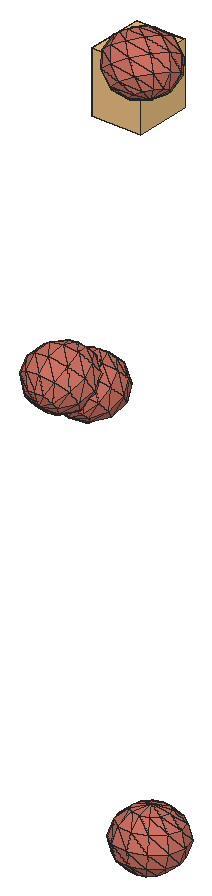
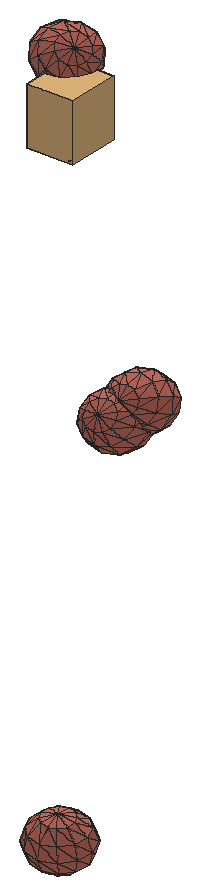
# SketchUp Ruby script. Lengths in inches.
U = 1.inch
M = Sketchup.active_model
def pt(a) = Geom::Point3d.new(a.map { |v| v * U })
def face(e, loops, mat)
  f = e.add_face(loops[0].map { |a| pt(a) })
  loops[1..].each { |l| e.add_face(l.map { |a| pt(a) }).erase! }
  f.material = f.back_material = mat if mat
  f
end
# faces: each face lists its corners as indices into pts; further lists are holes
def faces(e, pts, list, mat = nil) = list.each { |f| face(e, (f[0].is_a?(Array) ? f : [f]).map { |l| l.map { |i| pts[i] } }, mat) }
# xy, xz, yz: faces in a plane at the given z, y or x. An outline is a flat list of corners, or four numbers for a rectangle; further outlines are holes
def ring(l) = l.size == 4 ? [[l[0], l[1]], [l[2], l[1]], [l[2], l[3]], [l[0], l[3]]] : l.each_slice(2).to_a
def flat(e, list, mat, &to3) = list.each { |f| face(e, (f[0].is_a?(Array) ? f : [f]).map { |l| ring(l).map { |u, v| to3.(u, v) } }, mat) }
def xy(e, z, list, mat = nil) = flat(e, list, mat) { |x, y| [x, y, z] }
def xz(e, y, list, mat = nil) = flat(e, list, mat) { |x, z| [x, y, z] }
def yz(e, x, list, mat = nil) = flat(e, list, mat) { |y, z| [x, y, z] }
def lines(e, pts, list) = list.each { |a, b| e.add_line(pt(pts[a]), pt(pts[b])) }
# prism: a flat outline (further loops are holes) pulled along v
def prism(e, loops, v, mat = nil)
  f = face(e, loops, mat); d = Geom::Vector3d.new(v.map { |x| x * U })
  f.pushpull(f.normal.samedirection?(d) ? d.length : -d.length)
end
def box(e, o, s, mat = nil) = prism(e, [[o, [o[0] + s[0], o[1], o[2]], [o[0] + s[0], o[1] + s[1], o[2]], [o[0], o[1] + s[1], o[2]]]], [0, 0, s[2]], mat)
def at(x, y, z, deg = 0) = Geom::Transformation.translation(pt([x, y, z])) * Geom::Transformation.rotation(ORIGIN, Z_AXIS, deg.degrees)
def axes(o, x, y, z) = Geom::Transformation.new([*x, 0, *y, 0, *z, 0, *pt(o).to_a, 1])
def part(name) = M.definitions.add(name)
# library, detail: a bought-in or finely detailed component or shape, given as its bounding box
def library(name, o, s) = part(name).tap { |d| box(d.entities, o, s) }
def detail(e, o, s) = box(e.add_group.entities, o, s)
def put(e, d, t, mat = nil) = e.add_instance(d, t).tap { |i| i.material = mat if mat }
def group(e, t, mat = nil) = e.add_group.tap { |g| g.transformation = t; g.material = mat if mat }.entities
root = M.entities
M.materials.add("green").color = [174, 139, 102]
M.materials.add("vio").color = [206, 114, 100]
c1 = part("3DGeom~194_Defintion")
p = [[111.52,-262.8,-376.52],[-124.92,-186.52,-431.46],[-6.51,0,-500],[214.07,-101.27,-435.87],[-225.34,101.27,-430.15],[113.66,186.52,-434.56],
  [-121.28,262.8,-373.49],[318.08,-268.67,-220.68],[318.08,-268.67,-220.68],[377.29,-175.41,-254.95],[377.29,-175.41,-254.95],[318.13,60.26,-379.2],
  [318.13,60.26,-379.2],[318.13,60.26,-379.2],[203.36,323.0625,-252.6875],[-43.59,381.05,-215.98],[-43.59,381.05,-215.98],[203.36,323.0625,-252.6875],
  [37.95,-381.05,-217.04],[-209.87,-323.0625,-247.3125],[37.95,-381.05,-217.04],[-327.89,-60.26,-370.8],[-327.89,-60.26,-370.8],[-383.79,175.41,-245.05],
  [-225.34,101.27,-430.15],[-383.79,175.41,-245.05],[-323.71,268.67,-212.33],[-323.71,268.67,-212.33],[377.29,-175.41,-254.95],[318.13,60.26,-379.2],
  [437.37,-82.15,-222.23],[437.37,-82.15,-222.23],[318.13,60.26,-379.2],[395.82,178.51,-221.69],[318.13,60.26,-379.2],[203.36,323.0625,-252.6875],
  [395.82,178.51,-221.69],[275.6,-336.9375,-128.61],[37.95,-381.05,-217.04],[111.52,-262.8,-376.52],[275.6,-336.9375,-128.61],[111.52,-262.8,-376.52],
  [318.08,-268.67,-220.68],[-121.28,262.8,-373.49],[-323.71,268.67,-212.33],[-278.86,336.9375,-121.39],[-121.28,262.8,-373.49],[-43.59,381.05,-215.98],
  [-401.46,-178.51,-211.32],[-401.46,-178.51,-211.32],[-443,82.15,-210.78],[-327.89,-60.26,-370.8],[-327.89,-60.26,-370.8],[-383.79,175.41,-245.05],
  [318.08,-268.67,-220.68],[377.29,-175.41,-254.95],[439.41,-202.54,-5.72],[203.36,323.0625,-252.6875],[238.58,373.04,-3.1],[203.36,323.0625,-252.6875],
  [-13.09,424.33,0.17],[203.36,323.0625,-252.6875],[238.58,373.04,-3.1],[13.09,-424.33,-0.17],[-238.58,-373.04,3.1],[-209.87,-323.0625,-247.3125],
  [-209.87,-323.0625,-247.3125],[-238.58,-373.04,3.1],[-401.46,-178.51,-211.32],[-209.87,-323.0625,-247.3125],[-383.79,175.41,-245.05],[-439.41,202.54,5.72],
  [-323.71,268.67,-212.33],[-383.79,175.41,-245.05],[482.22,-13.88,-131.3],[426.32,221.79,-5.55],[275.6,-336.9375,-128.61],[261.25,-361.93,-3.4],
  [261.25,-361.93,-3.4],[275.6,-336.9375,-128.61],[-261.25,361.93,3.4],[-278.86,336.9375,-121.39],[-323.71,268.67,-212.33],[-238.58,-373.04,3.1],
  [-426.32,-221.79,5.55],[-401.46,-178.51,-211.32],[-485.47,13.88,-118.7],[-401.46,-178.51,-211.32],[-401.46,-178.51,-211.32],[499.83,11.11,-6.5],
  [261.25,-361.93,-3.4],[-261.25,361.93,3.4],[-278.86,336.9375,-121.39],[-499.83,-11.11,6.5],[485.47,-13.88,118.7],[401.46,178.51,211.32],
  [278.86,-336.9375,121.39],[323.71,-268.67,212.33],[383.79,-175.41,245.05],[443,-82.15,210.78],[209.87,323.0625,247.3125],[209.87,323.0625,247.3125],
  [278.86,-336.9375,121.39],[261.25,-361.93,-3.4],[238.58,373.04,-3.1],[-37.95,381.05,217.04],[209.87,323.0625,247.3125],[238.58,373.04,-3.1],
  [-37.95,381.05,217.04],[43.59,-381.05,215.98],[278.86,-336.9375,121.39],[-275.6,336.9375,128.61],[-37.95,381.05,217.04],[-203.36,-323.0625,252.6875],
  [-203.36,-323.0625,252.6875],[-238.58,-373.04,3.1],[-275.6,336.9375,128.61],[-261.25,361.93,3.4],[-203.36,-323.0625,252.6875],[-395.82,-178.51,221.69],
  [-482.22,13.88,131.3],[-437.37,82.15,222.23],[-377.29,175.41,254.95],[-377.29,175.41,254.95],[-318.08,268.67,220.68],[-318.08,268.67,220.68],
  [-275.6,336.9375,128.61],[327.89,60.26,370.8],[323.71,-268.67,212.33],[278.86,-336.9375,121.39],[-37.95,381.05,217.04],[-318.08,268.67,220.68],
  [-318.13,-60.26,379.2],[-318.13,-60.26,379.2],[225.34,-101.27,430.15],[225.34,-101.27,430.15],[401.46,178.51,211.32],[124.92,186.52,431.46],
  [327.89,60.26,370.8],[401.46,178.51,211.32],[209.87,323.0625,247.3125],[323.71,-268.67,212.33],[121.28,-262.8,373.49],[383.79,-175.41,245.05],
  [121.28,-262.8,373.49],[323.71,-268.67,212.33],[121.28,-262.8,373.49],[-203.36,-323.0625,252.6875],[43.59,-381.05,215.98],[-37.95,381.05,217.04],
  [-318.08,268.67,220.68],[-111.52,262.8,376.51],[-37.95,381.05,217.04],[-111.52,262.8,376.51],[-318.08,268.67,220.68],[-377.29,175.41,254.95],
  [-113.66,-186.52,434.56],[-395.82,-178.51,221.69],[-203.36,-323.0625,252.6875],[-318.13,-60.26,379.2],[-395.82,-178.51,221.69],[-214.07,101.27,435.87],
  [-437.37,82.15,222.23],[-437.37,82.15,222.23],[383.79,-175.41,245.05],[225.34,-101.27,430.15],[121.28,-262.8,373.49],[121.28,-262.8,373.49],
  [-203.36,-323.0625,252.6875],[327.89,60.26,370.8],[6.51,0,500],[327.89,60.26,370.8],[121.28,-262.8,373.49]]
faces(c1.entities,p,[[0,1,2],[0,2,3],[1,4,2],[3,2,5],[2,4,6],[2,6,5],[7,0,3],[8,3,9],
  [10,3,11],[3,5,12],[13,5,14],[5,6,15],[5,16,17],[18,19,1],[20,1,0],[19,21,1],
  [1,21,4],[22,23,24],[4,25,26],[4,27,6],[28,29,30],[31,32,33],[34,35,36],[37,38,39],
  [40,41,42],[43,44,45],[46,45,47],[19,48,21],[49,50,51],[52,50,53],[54,55,56],[55,31,56],
  [33,57,58],[59,47,60],[61,60,62],[63,64,65],[63,66,38],[67,68,69],[70,50,71],[72,73,71],
  [31,74,56],[31,33,74],[74,33,75],[33,58,75],[76,54,56],[77,63,38],[78,38,79],[47,45,80],
  [47,80,60],[81,82,71],[83,84,85],[84,86,87],[88,86,50],[50,86,71],[74,89,56],[74,75,89],
  [90,76,56],[91,92,71],[84,93,86],[86,93,71],[89,94,56],[89,95,94],[89,75,95],[96,90,56],
  [97,96,56],[98,97,56],[99,98,56],[94,99,56],[75,100,95],[75,58,101],[102,63,103],[104,105,106],
  [107,60,108],[109,64,63],[110,109,63],[60,80,111],[60,111,112],[109,113,64],[114,84,115],[116,117,71],
  [118,119,84],[119,93,84],[93,120,71],[120,121,71],[121,122,71],[123,124,71],[125,126,71],[119,120,93],
  [94,127,99],[94,95,127],[128,109,129],[130,111,131],[132,120,119],[133,121,120],[99,134,98],[99,127,135],
  [136,137,138],[139,140,137],[141,142,109],[143,144,145],[146,147,148],[149,150,151],[140,152,153],[153,154,155],
  [156,157,158],[156,159,160],[161,162,159],[161,155,163],[164,165,166],[140,153,137],[167,156,168],[153,155,161],
  [169,170,165],[171,137,170],[165,156,172],[137,153,161],[170,159,156],[170,161,159],[165,170,156],[137,161,170]],"vio")
c2 = part("3DGeom~189_Defintion")
p = [[117.375,12.85,-489.11],[33.19,-268.35,-390.125],[-76.27,-85.37,-487.14],[256.79,-154.93,-392.4],[251.43,147.02,-400.02],[-53.49,177.1875,-454.76],
  [23.91,254.65,-403.32],[-199.3,-309.86,-283.32],[-277.61,-121.32,-394.64],[-165.29,120.48,-453.62],[-210.02,294.05,-298.55],[-281.54,99.72,-400.21],
  [46.16,332.12,-313.1],[-281.54,99.72,-400.21],[-277.61,-121.32,-394.64],[-432.71,-85.37,-236.39],[-281.54,99.72,-400.21],[-371.08,120.48,-308.85],
  [-371.08,120.48,-308.85],[411.58,0,-289.54],[289.98,281.2,-243.75],[411.58,0,-289.54],[251.43,147.02,-400.02],[289.98,281.2,-243.75],
  [-277.61,-121.32,-394.64],[-199.3,-309.86,-283.32],[-378.39,-268.35,-100.59],[-277.61,-121.32,-394.64],[133.75,-379.42,-188.58],[327.4,-281.2,-190.55],
  [133.75,-379.42,-188.58],[411.58,0,-289.54],[327.4,-281.2,-190.55],[256.79,-154.93,-392.4],[33.19,-268.35,-390.125],[-67.59,-415.375,-96.08],
  [-199.3,-309.86,-283.32],[33.19,-268.35,-390.125],[133.75,-379.42,-188.58],[7.3125,388.83,-208.26],[289.98,281.2,-243.75],[46.16,332.12,-313.1],
  [46.16,332.12,-313.1],[-210.02,294.05,-298.55],[-500,12.85,-54.8],[-409.93,177.1875,-204.01],[-210.02,294.05,-298.55],[-387.68,254.65,-113.79],
  [-210.02,294.05,-298.55],[-387.68,254.65,-113.79],[-310.28,332.12,-62.35],[-210.02,294.05,-298.55],[-198.48,388.83,-63.49],[-210.02,294.05,-298.55],
  [-82.23,409.58,-116.9],[-210.02,294.05,-298.55],[-210.02,294.05,-298.55],[411.58,0,-289.54],[461.45,-147.02,-101.47],[327.4,-281.2,-190.55],
  [456.09,154.93,-109.09],[411.58,0,-289.54],[289.98,281.2,-243.75],[411.58,0,-289.54],[-199.3,-309.86,-283.32],[-222.6875,-379.42,62.16],
  [-199.3,-309.86,-283.32],[-222.6875,-379.42,62.16],[-378.39,-268.35,-100.59],[222.6875,379.42,-62.16],[289.98,281.2,-243.75],[222.6875,379.42,-62.16],
  [289.98,281.2,-243.75],[-456.09,-154.93,109.09],[-461.45,147.02,101.47],[-387.68,254.65,-113.79],[327.4,-281.2,-190.55],[198.48,-388.83,63.49],
  [327.4,-281.2,-190.55],[310.28,-332.12,62.35],[310.28,-332.12,62.35],[327.4,-281.2,-190.55],[82.23,-409.58,116.9],[67.59,415.375,96.08],
  [-387.68,254.65,-113.79],[-327.4,281.2,190.55],[-387.68,254.65,-113.79],[-327.4,281.2,190.55],[-310.28,332.12,-62.35],[500,-12.85,54.8],
  [378.39,268.35,100.59],[222.6875,379.42,-62.16],[387.68,-254.65,113.79],[310.28,-332.12,62.35],[-222.6875,-379.42,62.16],[-289.98,-281.2,243.75],
  [-7.3125,-388.83,208.26],[-222.6875,-379.42,62.16],[-133.75,379.42,188.58],[-327.4,281.2,190.55],[378.39,268.35,100.59],[-411.58,0,289.54],
  [409.93,-177.1875,204.01],[432.71,85.37,236.39],[-222.6875,-379.42,62.16],[-46.16,-332.12,313.1],[-222.6875,-379.42,62.16],[-46.16,-332.12,313.1],
  [-289.98,-281.2,243.75],[210.02,-294.05,298.55],[387.68,-254.65,113.79],[199.3,309.86,283.32],[378.39,268.35,100.59],[199.3,309.86,283.32],
  [-256.79,154.93,392.4],[-256.79,154.93,392.4],[-327.4,281.2,190.55],[-251.43,-147.02,400.02],[-251.43,-147.02,400.02],[210.02,-294.05,298.55],
  [-327.4,281.2,190.55],[-33.19,268.35,390.13],[-133.75,379.42,188.58],[-33.19,268.35,390.13],[-327.4,281.2,190.55],[-256.79,154.93,392.4],
  [-33.19,268.35,390.13],[371.08,-120.48,308.85],[210.02,-294.05,298.55],[-46.16,-332.12,313.1],[277.61,121.32,394.64],[199.3,309.86,283.32],
  [-289.98,-281.2,243.75],[-46.16,-332.12,313.1],[-23.91,-254.65,403.32],[-289.98,-281.2,243.75],[-251.43,-147.02,400.02],[-33.19,268.35,390.13],
  [277.61,121.32,394.64],[199.3,309.86,283.32],[-411.58,0,289.54],[-117.375,-12.85,489.11],[-411.58,0,289.54],[210.02,-294.05,298.55],
  [53.49,-177.1875,454.76],[210.02,-294.05,298.55],[165.29,-120.48,453.62],[210.02,-294.05,298.55],[281.54,-99.72,400.21],[210.02,-294.05,298.55],
  [371.08,-120.48,308.85],[281.54,-99.72,400.21],[210.02,-294.05,298.55],[281.54,-99.72,400.21],[76.27,85.37,487.14],[-33.19,268.35,390.13],
  [-33.19,268.35,390.13],[277.61,121.32,394.64],[281.54,-99.72,400.21],[277.61,121.32,394.64],[281.54,-99.72,400.21]]
faces(c2.entities,p,[[0,1,2],[0,3,1],[4,3,0],[5,0,2],[6,0,5],[6,4,0],[2,7,8],[2,1,7],
  [9,2,8],[5,2,9],[5,9,10],[6,5,10],[9,8,11],[9,11,10],[12,4,6],[12,6,10],
  [13,14,15],[16,15,17],[11,18,10],[4,19,3],[20,21,22],[12,23,4],[24,25,26],[27,26,15],
  [3,28,1],[3,29,30],[31,32,33],[34,35,36],[37,38,35],[39,40,41],[39,42,43],[17,15,44],
  [17,44,45],[17,45,46],[45,47,48],[49,50,51],[50,52,53],[54,39,55],[52,54,56],[57,58,59],
  [60,58,61],[62,60,63],[64,35,65],[66,67,68],[69,60,70],[39,71,72],[15,26,73],[15,73,44],
  [54,71,39],[45,44,74],[45,74,75],[76,77,38],[78,79,77],[58,80,81],[38,82,35],[38,77,82],
  [54,83,71],[52,83,54],[84,74,85],[86,87,88],[60,89,58],[90,89,60],[91,90,60],[58,92,93],
  [89,92,58],[26,94,95],[26,95,73],[35,96,97],[35,82,96],[50,98,52],[52,98,83],[50,99,98],
  [83,100,71],[44,73,101],[44,101,74],[89,102,92],[103,102,89],[90,103,89],[104,96,105],[106,107,108],
  [77,79,109],[79,110,109],[82,77,109],[83,111,112],[98,111,83],[113,103,90],[74,101,114],[74,115,116],
  [73,95,117],[73,118,101],[92,102,119],[96,82,109],[120,121,122],[98,123,111],[124,125,126],[102,127,128],
  [103,127,102],[129,96,109],[130,127,103],[131,130,103],[132,133,134],[135,134,136],[137,138,139],[140,136,141],
  [142,141,125],[134,133,143],[144,134,145],[146,144,147],[148,146,149],[150,151,152],[130,153,127],[125,154,155],
  [156,154,157],[125,141,154],[154,158,159],[136,134,144],[136,144,141],[154,146,160],[141,144,146],[141,146,154]],"vio")
c3 = part("3DGeom~224_Defintion")
p = [[81.72,-275.8,-371.94],[-133.11,-167.42,-440.41],[24.02,0,-500],[217.8,-130.81,-423.55],[-176.2,130.81,-442.48],[217.8,-130.81,-423.55],
  [174.72,167.42,-425.62],[-45.69,275.8,-378.0625],[-312.28,-14.1875,-390.87],[-329.21,226.5625,-266.39],[-253.86,310.28,-229.2],[-253.86,310.28,-229.2],
  [-23.47,-381.94,-218.13],[-254.58,-289.99,-262.81],[-23.47,-381.94,-218.13],[217.8,-130.81,-423.55],[348.3125,14.1875,-359.13],[348.3125,14.1875,-359.13],
  [278.6,289.99,-237.19],[44.27,381.94,-214.88],[44.27,381.94,-214.88],[278.6,289.99,-237.19],[274.66,-310.28,-203.8125],[217.8,-130.81,-423.55],
  [274.66,-310.28,-203.8125],[217.8,-130.81,-423.55],[353.23,-226.5625,-233.61],[353.23,-226.5625,-233.61],[217.8,-130.81,-423.55],[348.3125,14.1875,-359.13],
  [-417.47,-120.33,-237.0625],[-417.47,-120.33,-237.0625],[-407.77,142.85,-236.59],[-312.28,-14.1875,-390.87],[-407.77,142.85,-236.59],[-45.69,275.8,-378.0625],
  [-253.86,310.28,-229.2],[-201.92,371.56,-134.99],[-45.69,275.8,-378.0625],[44.27,381.94,-214.88],[213.93,-371.56,-115.01],[-23.47,-381.94,-218.13],
  [81.72,-275.8,-371.94],[213.93,-371.56,-115.01],[81.72,-275.8,-371.94],[274.66,-310.28,-203.8125],[428.58,-142.85,-196.42],[438.28,120.33,-195.95],
  [348.3125,14.1875,-359.13],[278.6,289.99,-237.19],[438.28,120.33,-195.95],[-329.21,226.5625,-266.39],[-407.77,142.85,-236.59],[-394.01,261.61,-18.93],
  [-253.86,310.28,-229.2],[-329.21,226.5625,-266.39],[-69.59,-420.79,-3.34],[-307.83,-334.85,-14.79],[-254.58,-289.99,-262.81],[-254.58,-289.99,-262.81],
  [-307.83,-334.85,-14.79],[-417.47,-120.33,-237.0625],[-254.58,-289.99,-262.81],[278.6,289.99,-237.19],[307.83,334.85,14.79],[278.6,289.99,-237.19],
  [69.59,420.79,3.34],[278.6,289.99,-237.19],[307.83,334.85,14.79],[-307.83,-334.85,-14.79],[-463.59,-159.18,-22.27],[-417.47,-120.33,-237.0625],
  [-468.51,81.57,-147.8],[-417.47,-120.33,-237.0625],[-417.47,-120.33,-237.0625],[-407.77,142.85,-236.59],[-407.77,142.85,-236.59],[274.66,-310.28,-203.8125],
  [394.01,-261.61,18.93],[394.01,-261.61,18.93],[-201.92,371.56,-134.99],[-253.86,310.28,-229.2],[187.3,-393.99,9],[213.93,-371.56,-115.01],
  [-187.3,393.99,-9],[213.93,-371.56,-115.01],[394.01,-261.61,18.93],[480.52,-81.57,-102.2],[394.01,-261.61,18.93],[463.59,159.18,22.27],
  [-495.13,59.14,-23.79],[-394.01,261.61,-18.93],[213.93,-371.56,-115.01],[394.01,-261.61,18.93],[495.13,-59.14,23.79],[394.01,-261.61,18.93],
  [-438.28,-120.33,195.95],[-480.52,81.57,102.2],[-278.6,-289.99,237.19],[-307.83,-334.85,-14.79],[-278.6,-289.99,237.19],[-428.58,142.85,196.42],
  [-353.23,226.5625,233.61],[-274.66,310.28,203.8125],[-274.66,310.28,203.8125],[-213.93,371.56,115.01],[-213.93,371.56,115.01],[-394.01,261.61,-18.93],
  [-44.27,-381.94,214.88],[-278.6,-289.99,237.19],[201.92,-371.56,134.99],[307.83,334.85,14.79],[23.47,381.94,218.13],[23.47,381.94,218.13],
  [254.58,289.99,262.81],[307.83,334.85,14.79],[23.47,381.94,218.13],[254.58,289.99,262.81],[253.86,-310.28,229.2],[201.92,-371.56,134.99],
  [394.01,-261.61,18.93],[329.21,-226.5625,266.39],[394.01,-261.61,18.93],[407.77,-142.85,236.59],[394.01,-261.61,18.93],[468.51,-81.57,147.8],
  [394.01,-261.61,18.93],[394.01,-261.61,18.93],[417.47,120.33,237.0625],[254.58,289.99,262.81],[-348.3125,-14.1875,359.13],[-348.3125,-14.1875,359.13],
  [23.47,381.94,218.13],[-274.66,310.28,203.8125],[253.86,-310.28,229.2],[312.28,14.1875,390.87],[312.28,14.1875,390.87],[-174.72,-167.42,425.62],
  [-438.28,-120.33,195.95],[-278.6,-289.99,237.19],[-348.3125,-14.1875,359.13],[-438.28,-120.33,195.95],[-217.8,130.81,423.55],[-348.3125,-14.1875,359.13],
  [-217.8,130.81,423.55],[-81.72,275.8,371.94],[-274.66,310.28,203.8125],[-353.23,226.5625,233.61],[23.47,381.94,218.13],[-274.66,310.28,203.8125],
  [-81.72,275.8,371.94],[45.69,-275.8,378.0625],[-278.6,-289.99,237.19],[-44.27,-381.94,214.88],[253.86,-310.28,229.2],[45.69,-275.8,378.0625],
  [254.58,289.99,262.81],[23.47,381.94,218.13],[329.21,-226.5625,266.39],[45.69,-275.8,378.0625],[253.86,-310.28,229.2],[-353.23,226.5625,233.61],
  [-217.8,130.81,423.55],[407.77,-142.85,236.59],[176.2,-130.81,442.48],[329.21,-226.5625,266.39],[407.77,-142.85,236.59],[312.28,14.1875,390.87],
  [417.47,120.33,237.0625],[133.11,167.42,440.41],[417.47,120.33,237.0625],[45.69,-275.8,378.0625],[-278.6,-289.99,237.19],[329.21,-226.5625,266.39],
  [45.69,-275.8,378.0625],[-24.02,0,500],[45.69,-275.8,378.0625]]
faces(c3.entities,p,[[0,1,2],[0,2,3],[1,4,2],[5,2,6],[2,4,7],[2,7,6],[1,8,4],[8,9,4],
  [4,9,10],[4,11,7],[12,13,1],[14,1,0],[13,8,1],[15,6,16],[17,6,18],[6,7,19],
  [6,20,21],[22,0,23],[24,25,26],[27,28,29],[13,30,8],[31,32,33],[8,34,9],[35,36,37],
  [38,37,39],[40,41,42],[43,44,45],[27,29,46],[46,29,47],[48,49,50],[51,52,53],[54,55,53],
  [56,57,58],[56,59,41],[60,61,62],[47,63,64],[65,39,66],[67,66,68],[69,70,71],[70,72,73],
  [74,72,75],[76,72,53],[77,27,78],[27,46,79],[80,81,53],[82,56,41],[82,41,83],[39,37,84],
  [39,84,66],[85,77,86],[46,87,88],[46,47,87],[87,47,89],[47,64,89],[70,90,72],[72,90,53],
  [84,37,91],[82,92,93],[87,94,95],[87,89,94],[96,90,70],[96,97,90],[90,97,53],[98,70,99],
  [100,96,70],[97,101,53],[101,102,53],[102,103,53],[104,105,53],[106,84,107],[108,57,56],[108,109,57],
  [66,84,106],[110,108,56],[110,56,82],[111,66,112],[66,106,113],[110,82,93],[89,64,114],[115,116,117],
  [118,119,120],[121,118,122],[123,121,124],[125,123,126],[94,125,127],[94,89,128],[89,129,128],[94,128,125],
  [130,97,96],[131,101,97],[132,106,133],[134,108,110],[125,135,123],[125,128,136],[137,138,139],[137,140,141],
  [142,101,143],[144,102,101],[145,146,147],[148,149,150],[151,152,153],[154,155,108],[156,157,145],[158,159,160],
  [145,161,162],[163,164,165],[166,167,164],[168,169,167],[170,156,169],[171,137,172],[156,145,169],[173,164,174],
  [175,140,137],[175,162,140],[169,145,162],[164,137,176],[167,175,164],[167,169,175],[169,162,175],[164,175,137]],"vio")
c4 = library("3DGeom~9_Defintion",[-447.05,-500,-392.82],[894.1,1000,785.64])
c5 = part("3DGeom~10_Defintion")
p = [[-376.65,-477.04,-383.86],[-408.2,-455.37,-392.67],[-389.75,-464.73,-392.82],[-376.65,-477.04,-383.86],[-442.82,-474.42,-333.72],[-408.2,-455.37,-392.67],
  [-408.2,-455.37,-392.67],[-442.82,-474.42,-333.72],[-441.29,-454.05,-367.6],[-408.2,-455.37,-392.67],[-441.29,-454.05,-367.6],[-427.07,-451.46,-383.43],
  [-378.18,-497.41,-349.98],[-442.82,-474.42,-333.72],[-376.65,-477.04,-383.86],[-378.18,-497.41,-349.98],[-376.65,-477.04,-383.86],[-372.41,-489,-368.18],
  [-442.82,-474.42,-333.72],[-447.05,-462.46,-349.4],[-441.29,-454.05,-367.6],[-411.26,-496.09,-324.91],[-378.18,-497.41,-349.98],[-392.4,-500,-334.15],
  [-411.26,-496.09,-324.91],[-442.82,-474.42,-333.72],[-378.18,-497.41,-349.98],[-442.82,-474.42,-333.72],[-411.26,-496.09,-324.91],[-429.72,-486.73,-324.76],
  [401.4,485.85,384.88],[441.04,458.37,319.44],[429.72,472.35,311.5],[401.4,485.85,384.88],[429.72,472.35,311.5],[416.12,486.26,314.46],
  [401.4,485.85,384.88],[416.12,486.26,314.46],[403.89,496.38,327.52],[401.4,485.85,384.88],[447.05,448.07,336.15],[441.04,458.37,319.44],
  [401.4,485.85,384.88],[403.89,496.38,327.52],[396.3,500,347.18],[401.4,485.85,384.88],[446.15,444.22,357.14],[447.05,448.07,336.15],
  [401.4,485.85,384.88],[396.3,500,347.18],[395.39,496.14,368.18],[401.4,485.85,384.88],[438.56,447.84,376.81],[446.15,444.22,357.14],
  [401.4,485.85,384.88],[426.33,457.96,389.87],[438.56,447.84,376.81],[401.4,485.85,384.88],[412.73,471.87,392.82],[426.33,457.96,389.87]]
faces(c5.entities,p,[[0,1,2],[3,4,5],[6,7,8],[9,10,11],[12,13,14],[15,16,17],[18,19,20],[21,22,23],
  [24,25,26],[27,28,29],[30,31,32],[33,34,35],[36,37,38],[39,40,41],[42,43,44],[45,46,47],
  [48,49,50],[51,52,53],[54,55,56],[57,58,59]],"green")
c6 = part("3DGeom~192_Defintion")
p = [[46.59,-12.33,-500],[-151.08,-242.85,-384.34],[-208.06,-36.06,-455.29],[69.45,-222.31,-423.06],[288.76,14.69,-410.73],[11.25,200.94,-442.97],
  [220.97,224.35,-365.66],[-323.33,-255.02,-239.97],[-406.96,-50.11,-288.59],[-323.33,-255.02,-239.97],[-209.29,180.4,-404.25],[-406.96,-50.11,-288.59],
  [-27.11,360.38,-267.25],[93.97,373.89,-222.61],[-27.11,360.38,-267.25],[93.97,373.89,-222.61],[-53.62,-384.57,-210.4],[73.7,-372.71,-232.75],
  [-53.62,-384.57,-210.4],[279.17,-198.9,-345.75],[453.55,37.78,-211.41],[279.17,-198.9,-345.75],[288.76,14.69,-410.73],[363.68,244.34,-193.04],
  [288.76,14.69,-410.73],[220.97,224.35,-365.66],[363.68,244.34,-193.04],[288.76,14.69,-410.73],[-406.96,-50.11,-288.59],[-381.54,168.23,-259.88],
  [-154.4375,348.52,-244.89],[-381.54,168.23,-259.88],[-27.11,360.38,-267.25],[-154.4375,348.52,-244.89],[-151.08,-242.85,-384.34],[-153.07,-391.6,-127.05],
  [-323.33,-255.02,-239.97],[-151.08,-242.85,-384.34],[-53.62,-384.57,-210.4],[176.37,385.43,-122.95],[220.97,224.35,-365.66],[93.97,373.89,-222.61],
  [363.68,244.34,-193.04],[220.97,224.35,-365.66],[194.79,-359.2,-188.12],[421.89,-178.91,-173.13],[194.79,-359.2,-188.12],[279.17,-198.9,-345.75],
  [279.17,-198.9,-345.75],[-406.96,-50.11,-288.59],[-401.15,-255.57,-28.63],[-496.8125,-50.74,-44.56],[-323.33,-255.02,-239.97],[-381.54,168.23,-259.88],
  [-27.11,360.38,-267.25],[-154.4375,348.52,-244.89],[-58.21,423.25,-19.91],[-459.36,167.68,-48.54],[-253.89,341.49,-161.54],[-154.4375,348.52,-244.89],
  [-381.54,168.23,-259.88],[-253.89,341.49,-161.54],[-253.89,341.49,-161.54],[-323.33,-255.02,-239.97],[-198,-391.92,-5.03],[-401.15,-255.57,-28.63],
  [-323.33,-255.02,-239.97],[73.7,-372.71,-232.75],[58.21,-423.25,19.91],[73.7,-372.71,-232.75],[194.79,-359.2,-188.12],[496.8125,50.74,44.56],
  [401.15,255.57,28.63],[363.68,244.34,-193.04],[401.15,255.57,28.63],[198,391.92,5.03],[401.15,255.57,28.63],[194.79,-359.2,-188.12],
  [277.18,-347.66,-88.46],[277.18,-347.66,-88.46],[194.79,-359.2,-188.12],[459.36,-167.68,48.55],[-253.89,341.49,-161.54],[-298.81,341.17,-39.53],
  [-298.81,341.17,-39.53],[277.18,-347.66,-88.46],[298.81,-341.17,39.53],[298.81,-341.17,39.53],[-453.55,-37.78,211.41],[-421.89,178.91,173.13],
  [-298.81,341.17,-39.53],[-363.68,-244.34,193.05],[-298.81,341.17,-39.53],[-277.18,347.66,88.46],[-277.18,347.66,88.46],[-401.15,-255.57,-28.63],
  [-176.37,-385.43,122.95],[-401.15,-255.57,-28.63],[-363.68,-244.34,193.05],[-194.79,359.2,188.12],[-73.7,372.71,232.75],[53.62,384.57,210.4],
  [153.07,391.6,127.05],[-93.97,-373.89,222.61],[27.11,-360.38,267.25],[-93.97,-373.89,222.61],[154.4375,-348.52,244.89],[27.11,-360.38,267.25],
  [298.81,-341.17,39.53],[253.89,-341.49,161.54],[253.89,-341.49,161.54],[154.4375,-348.52,244.89],[323.33,255.02,239.97],[401.15,255.57,28.63],
  [323.33,255.02,239.97],[381.54,-168.23,259.88],[253.89,-341.49,161.54],[406.96,50.11,288.59],[323.33,255.02,239.97],[-277.18,347.66,88.46],
  [-279.17,198.9,345.75],[-277.18,347.66,88.46],[-279.17,198.9,345.75],[-194.79,359.2,188.12],[-363.68,-244.34,193.05],[-93.97,-373.89,222.61],
  [209.29,-180.4,404.25],[154.4375,-348.52,244.89],[253.89,-341.49,161.54],[253.89,-341.49,161.54],[381.54,-168.23,259.88],[-288.76,-14.69,410.73],
  [-288.76,-14.69,410.73],[-279.17,198.9,345.75],[-194.79,359.2,188.12],[-279.17,198.9,345.75],[-69.45,222.31,423.06],[-194.79,359.2,188.12],
  [-73.7,372.71,232.75],[-363.68,-244.34,193.05],[-93.97,-373.89,222.61],[-220.97,-224.35,365.66],[-220.97,-224.35,365.66],[-73.7,372.71,232.75],
  [151.08,242.85,384.34],[53.62,384.57,210.4],[151.08,242.85,384.34],[-220.97,-224.35,365.66],[-288.76,-14.69,410.73],[-220.97,-224.35,365.66],
  [-93.97,-373.89,222.61],[27.11,-360.38,267.25],[-73.7,372.71,232.75],[151.08,242.85,384.34],[151.08,242.85,384.34],[406.96,50.11,288.59],
  [323.33,255.02,239.97],[-11.25,-200.94,442.97],[208.06,36.05,455.29],[381.54,-168.23,259.88],[381.54,-168.23,259.88],[406.96,50.11,288.59],
  [151.08,242.85,384.34],[406.96,50.11,288.59],[-288.76,-14.69,410.73],[-46.59,12.33,500],[151.08,242.85,384.34]]
faces(c6.entities,p,[[0,1,2],[0,3,1],[4,3,0],[5,0,2],[6,0,5],[6,4,0],[2,7,8],[2,1,9],
  [10,2,11],[5,2,10],[12,5,10],[13,5,14],[15,6,5],[3,16,1],[3,17,18],[19,17,3],
  [4,19,3],[20,21,22],[23,24,25],[26,20,27],[10,28,29],[30,10,31],[32,10,33],[34,35,36],
  [37,38,35],[39,40,41],[39,42,43],[19,44,17],[45,46,47],[20,45,48],[49,50,51],[49,52,50],
  [53,49,51],[54,55,56],[41,54,56],[53,51,57],[58,53,57],[59,60,61],[55,62,56],[63,64,65],
  [66,35,64],[38,67,68],[69,70,68],[39,41,56],[71,45,20],[72,20,73],[74,71,20],[35,38,68],
  [75,42,39],[75,76,42],[77,78,68],[45,79,80],[81,79,45],[71,81,45],[82,57,83],[62,84,56],
  [64,35,68],[75,39,56],[85,86,68],[81,87,79],[57,51,88],[57,88,89],[90,57,89],[51,50,91],
  [51,91,88],[92,89,93],[84,94,56],[95,64,96],[97,96,98],[94,99,56],[99,100,56],[100,101,56],
  [101,102,56],[102,75,56],[96,64,68],[102,76,75],[103,96,68],[104,105,68],[106,107,68],[108,109,68],
  [110,111,68],[112,71,113],[102,114,76],[115,116,87],[115,87,81],[117,81,71],[118,117,71],[117,115,81],
  [119,89,120],[121,122,123],[124,96,125],[101,114,102],[126,127,128],[126,129,130],[89,88,131],[89,132,133],
  [134,135,136],[137,136,138],[139,140,141],[88,91,142],[143,144,145],[101,146,114],[88,147,148],[149,150,151],
  [152,136,153],[154,155,156],[157,151,127],[157,127,126],[158,126,159],[158,160,161],[149,151,157],[162,158,163],
  [135,164,165],[135,165,136],[164,149,157],[136,158,166],[165,157,126],[165,126,158],[164,157,165],[136,165,158]],"vio")
g1 = group(root,at(15.3125,38.42,26.21))
put(g1,c1,axes([3.29,-0.23,13.07],[0,0.00039,0],[0,0,-0.00039],[-0.00039,0,0]),"vio")
g2 = group(root,at(15.3125,38.42,26.21))
put(g2,c2,axes([3.75,-0.22,14.87],[0,0.00039,0],[0,0,-0.00039],[-0.00039,0,0]),"vio")
g3 = group(root,at(15.3125,38.42,26.21))
put(g3,c3,axes([3.35,-0.11,13],[0,0.00039,0],[0,0,-0.00039],[-0.00039,0,0]),"vio")
g4 = group(root,at(15.3125,38.42,26.21))
put(g4,c4,axes([3.6,-0.06,14.67],[0,0.00036,0],[0,0,-0.00036],[-0.00036,0,0]),"green")
put(g4,c5,axes([3.6,-0.06,14.67],[0,0.00036,0],[0,0,-0.00036],[-0.00036,0,0]),"green")
g5 = group(root,at(15.3125,38.42,26.21))
put(g5,c6,axes([3.57,0.06,10.63],[0,0.00039,0],[0,0,-0.00039],[-0.00039,0,0]),"vio")
